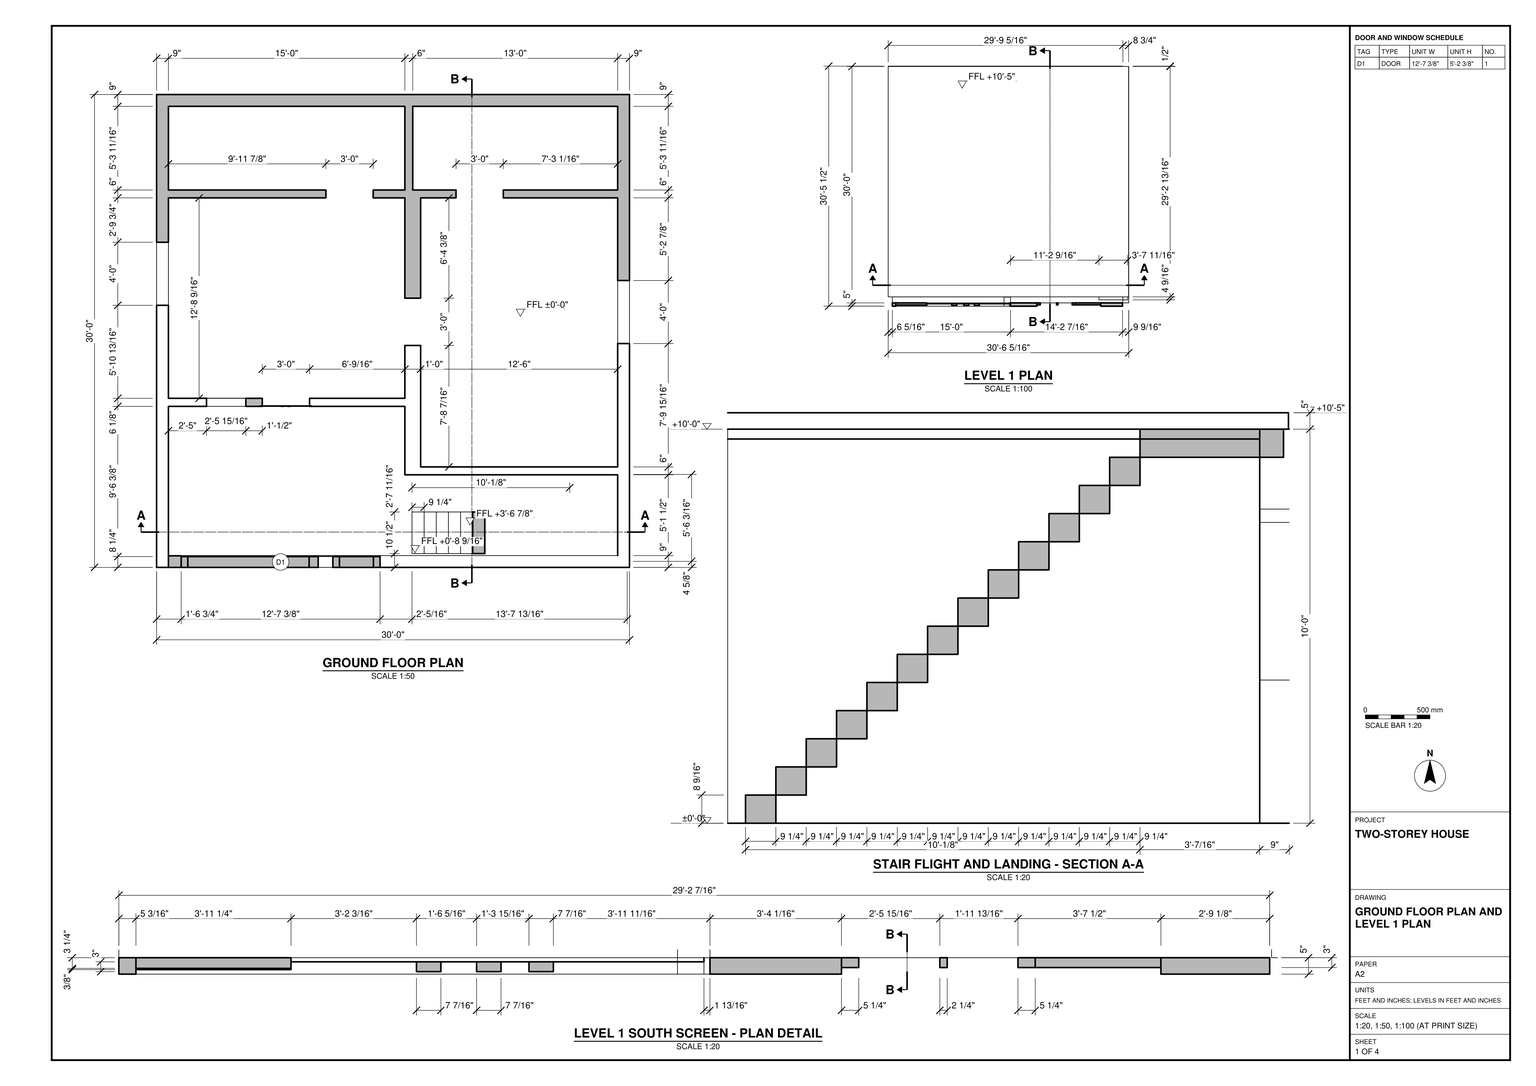
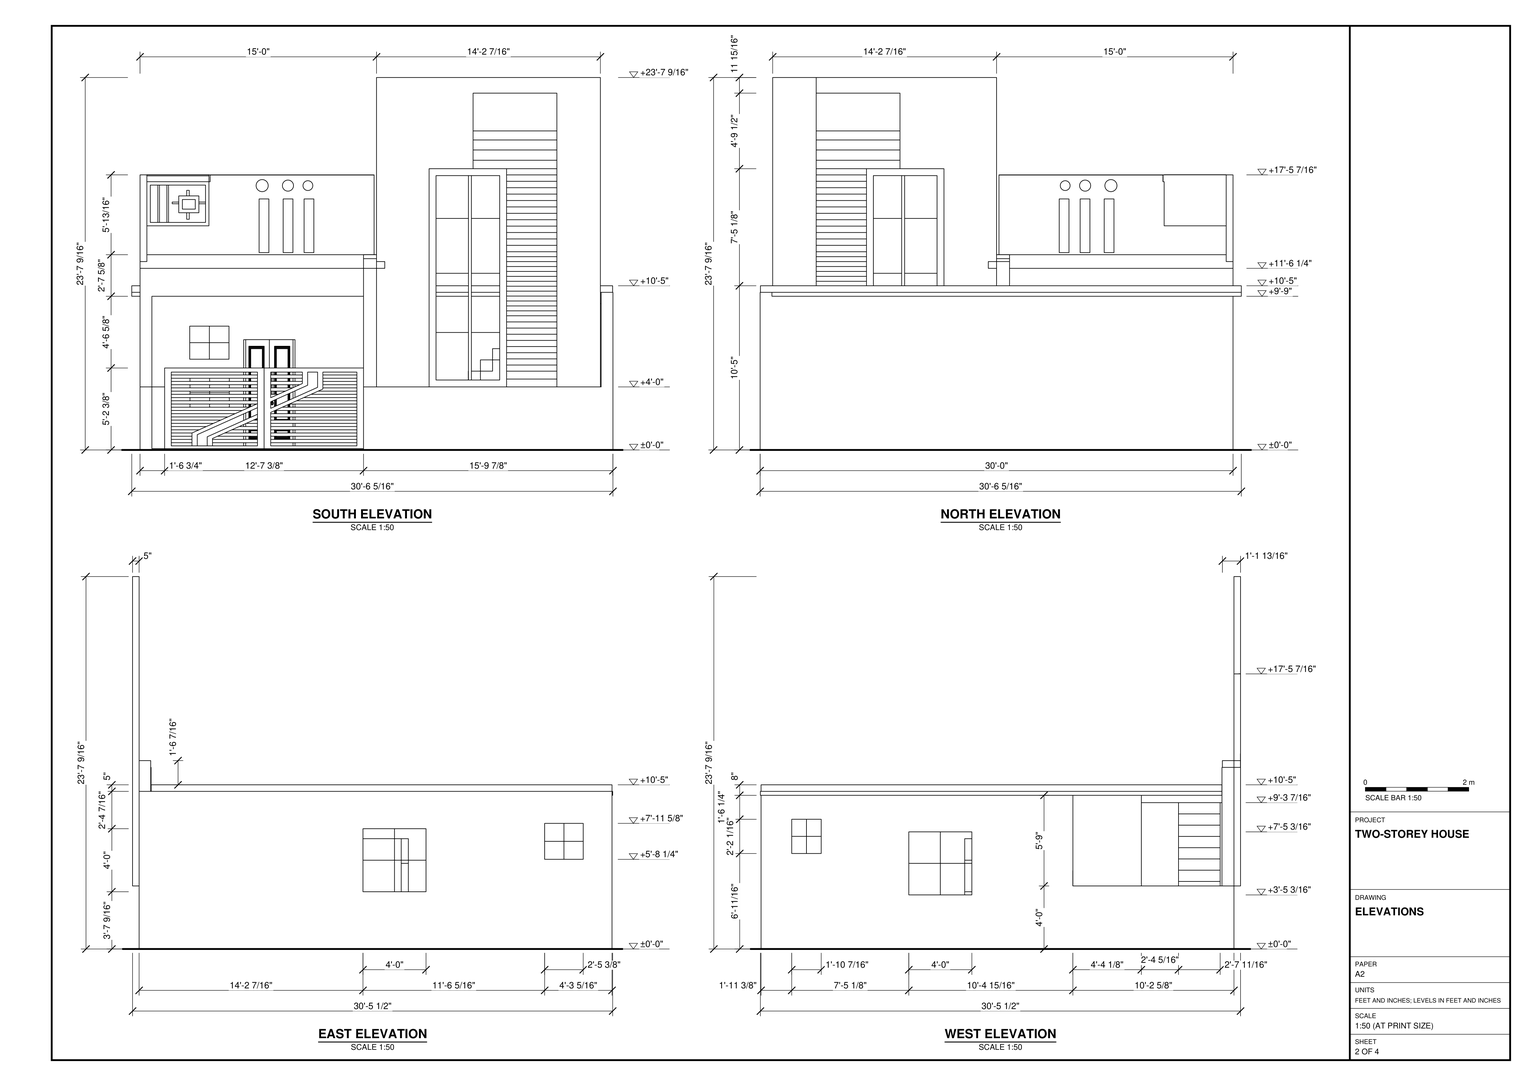
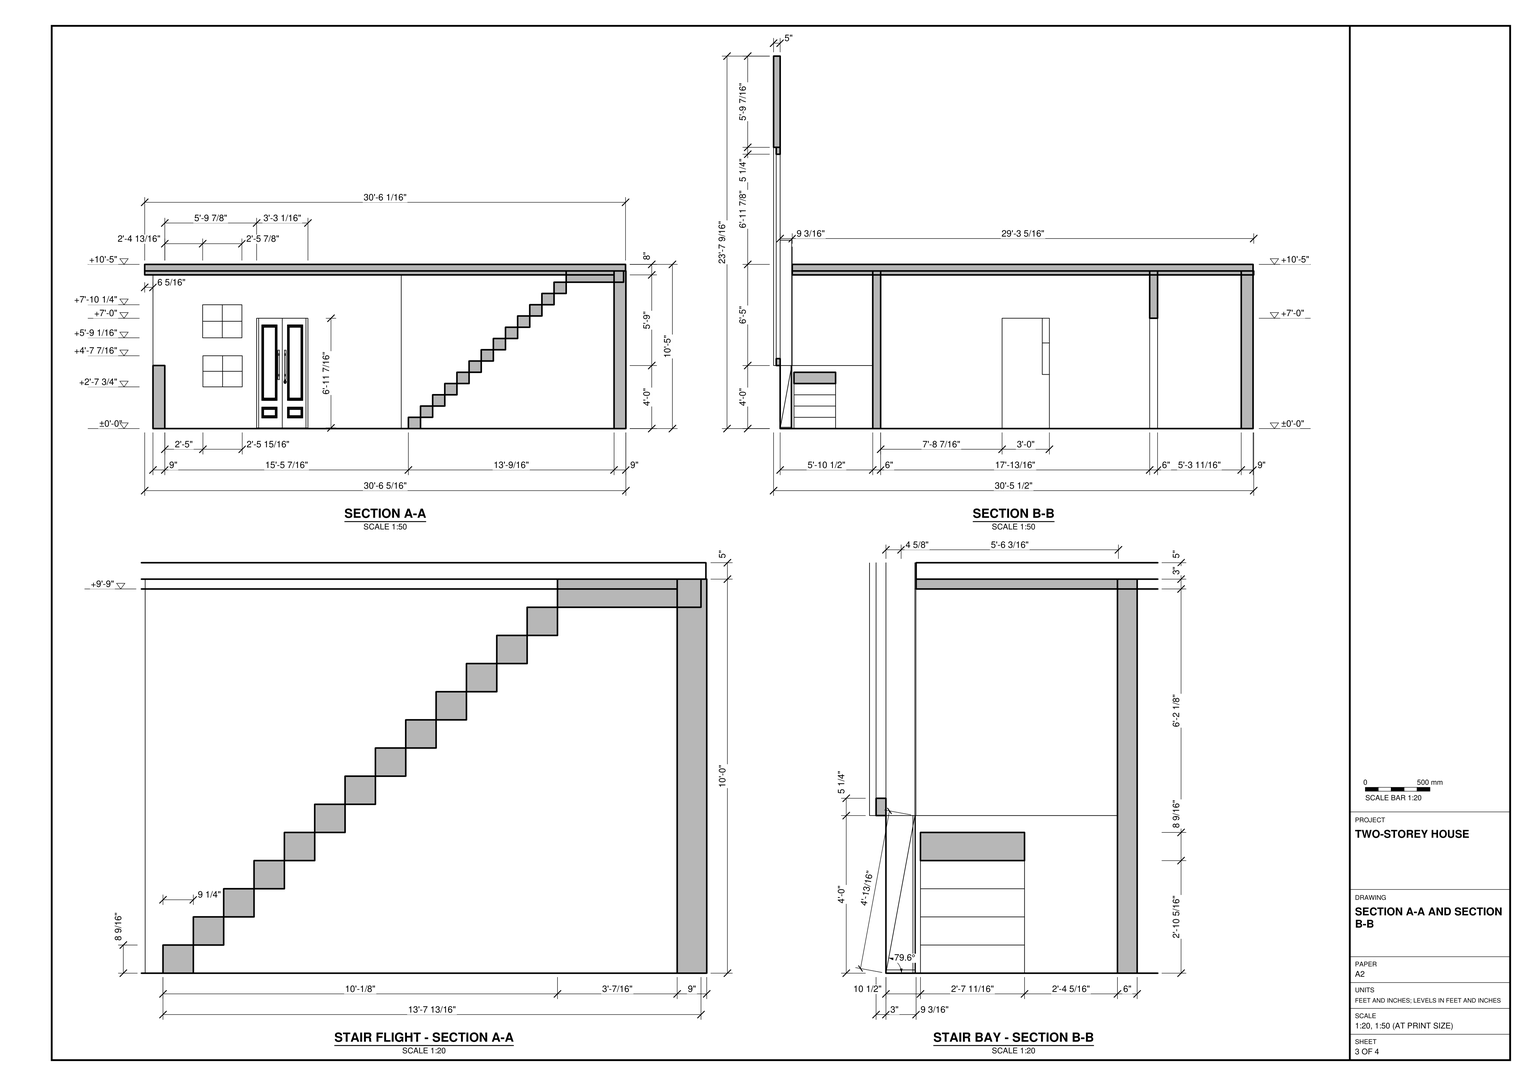
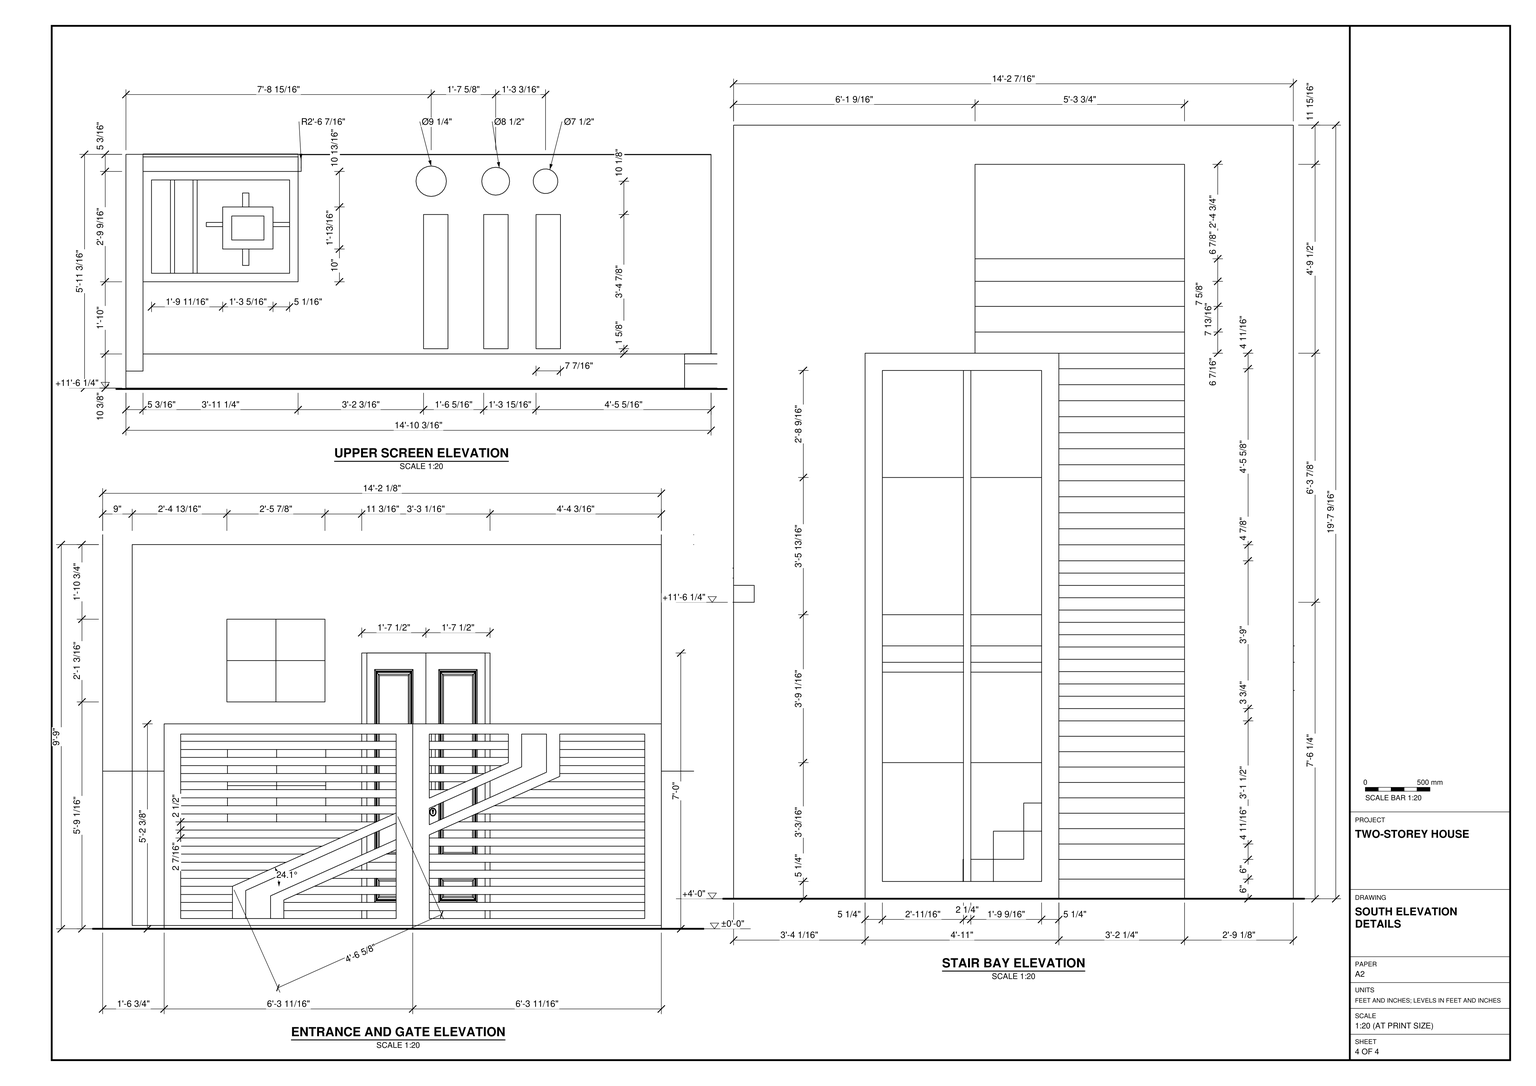
Build the house in SketchUp from task_files/diagram_01.pdf. Work in feet and inches. Orient the screened entrance toward the south. The overall model measures 30'-6 5/16" east to west, 30'-5 1/2" north to south and 23'-7 9/16" high. Set the ground floor at ±0'-0" and Level 1 at +10'-5".

Lay out the ground floor with the 9" exterior walls and 6" partitions shown in plan. Form the two rooms across the north end, the larger spaces south of them and the recessed entrance behind the front gate. Place the doorways and divided windows using the plan and elevations. Model the straight stair in the southeast bay, including its treads and upper landing. Use the sections to set the landing against the flat Level 1 slab and to shape the projecting slab edge.

Leave the upper slab open behind the south screen. Viewed from the south, the shorter panel sits over the gate on the left; the tall frame, horizontal bands and narrow divided panel stand on the right. Use the screen plan detail to place these elements at their different depths. Model the gate with its horizontal bars and diagonal motif.

Keep shell elements such as walls, slabs and roof, and each furniture or joinery piece shown, in separate groups or components; use components for repeated parts. Decor and loose items shown may be represented by any suitable library component. Save one SketchUp model as output_files/two_storey_house_with_a_stepped_south_screen.skp.

# SketchUp Ruby script. Lengths in inches.
U = 1.inch
M = Sketchup.active_model
def pt(a) = Geom::Point3d.new(a.map { |v| v * U })
def face(e, loops, mat)
  f = e.add_face(loops[0].map { |a| pt(a) })
  loops[1..].each { |l| e.add_face(l.map { |a| pt(a) }).erase! }
  f.material = f.back_material = mat if mat
  f
end
# faces: each face lists its corners as indices into pts; further lists are holes
def faces(e, pts, list, mat = nil) = list.each { |f| face(e, (f[0].is_a?(Array) ? f : [f]).map { |l| l.map { |i| pts[i] } }, mat) }
# xy, xz, yz: faces in a plane at the given z, y or x. An outline is a flat list of corners, or four numbers for a rectangle; further outlines are holes
def ring(l) = l.size == 4 ? [[l[0], l[1]], [l[2], l[1]], [l[2], l[3]], [l[0], l[3]]] : l.each_slice(2).to_a
def flat(e, list, mat, &to3) = list.each { |f| face(e, (f[0].is_a?(Array) ? f : [f]).map { |l| ring(l).map { |u, v| to3.(u, v) } }, mat) }
def xy(e, z, list, mat = nil) = flat(e, list, mat) { |x, y| [x, y, z] }
def xz(e, y, list, mat = nil) = flat(e, list, mat) { |x, z| [x, y, z] }
def yz(e, x, list, mat = nil) = flat(e, list, mat) { |y, z| [x, y, z] }
def lines(e, pts, list) = list.each { |a, b| e.add_line(pt(pts[a]), pt(pts[b])) }
# prism: a flat outline (further loops are holes) pulled along v
def prism(e, loops, v, mat = nil)
  f = face(e, loops, mat); d = Geom::Vector3d.new(v.map { |x| x * U })
  f.pushpull(f.normal.samedirection?(d) ? d.length : -d.length)
end
def box(e, o, s, mat = nil) = prism(e, [[o, [o[0] + s[0], o[1], o[2]], [o[0] + s[0], o[1] + s[1], o[2]], [o[0], o[1] + s[1], o[2]]]], [0, 0, s[2]], mat)
def at(x, y, z, deg = 0) = Geom::Transformation.translation(pt([x, y, z])) * Geom::Transformation.rotation(ORIGIN, Z_AXIS, deg.degrees)
def axes(o, x, y, z) = Geom::Transformation.new([*x, 0, *y, 0, *z, 0, *pt(o).to_a, 1])
def part(name) = M.definitions.add(name)
# library, detail: a bought-in or finely detailed component or shape, given as its bounding box
def library(name, o, s) = part(name).tap { |d| box(d.entities, o, s) }
def detail(e, o, s) = box(e.add_group.entities, o, s)
def put(e, d, t, mat = nil) = e.add_instance(d, t).tap { |i| i.material = mat if mat }
def group(e, t, mat = nil) = e.add_group.tap { |g| g.transformation = t; g.material = mat if mat }.entities
root = M.entities
M.materials.add("[Carrera Marble]").color = [207, 207, 207]
M.materials.add("[Color A08]").color = [102, 0, 0]
M.materials.add("[Color B04]").color = [255, 101, 50]
M.materials.add("[Color C06]").color = [204, 102, 0]
M.materials.add("[Color D06]").color = [204, 153, 0]
M.materials.add("[Color H06]").color = [0, 204, 204]
M.materials.add("[Color I02]").color = [153, 153, 255]
M.materials.add("[Color J02]").color = [204, 153, 255]
M.materials.add("[Color J03]").color = [178, 101, 255]
M.materials.add("[Color L02]").color = [255, 153, 204]
M.materials.add("[Color L04]").color = [255, 50, 152]
M.materials.add("[Color L11]").color = [153, 0, 76]
M.materials.add("[Color M04]").color = [142, 142, 142]
M.materials.add("[Color M06]").color = [86, 86, 86]
M.materials.add("[Color M08]").color = [30, 30, 30]
M.materials.add("[Concrete Aggregate Smoke]").color = [154, 150, 148]
M.materials.add("[Granite Light Gray]").color = [149, 148, 144]
M.materials.add("[Marble Carrara Gold Floor Tile]").color = [225, 223, 217]
M.materials.add("[Stone Vein Gray]").color = [166, 165, 165]
M.materials.add("[Translucent Glass Sky Reflection]").color = [126, 138, 183]
M.materials["[Translucent Glass Sky Reflection]"].alpha = 0.52
M.materials.add("[Wood Board Cork]").color = [215, 201, 115]
c1 = library("Modern+Gate+1",[-0.84,-7.98,-0.92],[117.88,7.98,57.34])
c2 = library("DD LT 2",[0,0,0],[47.24,4.7,78.74])
xy(root,0,[[[6.3125,5,6.3125,365,366.3125,365,366.3125,5,176.43,5,176.43,13.8125,25.03,13.8125,25.03,5],[15.3125,14,357.3125,14,357.3125,75.5,195.3125,75.5,195.3125,127.6,122.77,127.6,122.77,133.72,195.3125,133.72,195.3125,173.96,207.3125,173.96,207.3125,81.5,357.3125,81.5,357.3125,286.3125,270.25,286.3125,270.25,292.3125,357.3125,292.3125,357.3125,356,201.3125,356,201.3125,292.3125,234.25,292.3125,234.25,286.3125,207.3125,286.3125,207.3125,209.96,195.3125,209.96,195.3125,286.3125,171.2,286.3125,171.2,292.3125,195.3125,292.3125,195.3125,356,15.3125,356,15.3125,292.3125,135.2,292.3125,135.2,286.3125,15.3125,286.3125,15.3125,133.72,86.77,133.72,86.77,127.6,15.3125,127.6]],[25.03,5,176.43,13.8125]])
xy(root,0,[[15.3125,14,357.3125,14,357.3125,75.5,195.3125,75.5,195.3125,127.6,122.77,127.6,122.77,133.72,195.3125,133.72,195.3125,173.96,207.3125,173.96,207.3125,81.5,357.3125,81.5,357.3125,286.3125,270.25,286.3125,270.25,292.3125,357.3125,292.3125,357.3125,356,201.3125,356,201.3125,292.3125,234.25,292.3125,234.25,286.3125,207.3125,286.3125,207.3125,209.96,195.3125,209.96,195.3125,286.3125,171.2,286.3125,171.2,292.3125,195.3125,292.3125,195.3125,356,15.3125,356,15.3125,292.3125,135.2,292.3125,135.2,286.3125,15.3125,286.3125,15.3125,133.72,86.77,133.72,86.77,127.6,15.3125,127.6]],"[Marble Carrara Gold Floor Tile]")
xy(root,1,[[15.3125,5,25.03,13.8125],[25.03,5,176.43,13.8125]])
xy(root,31.75,[[44.32,127.6,74.26,133.72],[44.32,133.72,74.26,133.85]])
xy(root,41.19,[[6.3125,204.53,15.3125,252.53]])
xy(root,43.59,[[357.3125,175.41,366.3125,223.41]])
xy(root,48,[[186.3125,0,226.36,5],[323.625,0,356.75,5],[226.36,2,285.36,5],[285.36,2,323.625,5],[6.3125,5,15.3125,14.125],
  [15.3125,5,25.03,13.8125],[176.43,5,186.3125,13.8125]])
xy(root,48,[[6.3125,14.125,15.3125,127.6]],"[Color M08]")
xy(root,53.26,[[231.62,2,256.3,5],[256.3,2,258.55,5],[258.55,2,280.1,5]])
xy(root,53.97,[[285.36,2,323.625,5]],"[Color A08]")
xy(root,55.4375,[[44.32,127.6,74.26,133.72],[44.32,133.72,74.26,133.85]])
xy(root,59.97,[[285.36,5,323.625,8]])
xy(root,59.97,[[285.36,2,323.625,5]],"[Color A08]")
xy(root,64.66,[[285.36,5,323.625,8]])
xy(root,64.66,[[285.36,2,323.625,5]],"[Color A08]")
xy(root,68.28,[[357.3125,313.71,366.3125,343.08]])
xy(root,69.09,[[44.14,127.6,74.01,133.72]])
xy(root,69.35,[[285.36,2,323.625,5]],"[Color A08]")
xy(root,72.72,[[6.3125,319.21,15.3125,341.65]])
xy(root,74.04,[[285.36,2,323.625,5]],"[Color A08]")
xy(root,78.72,[[285.36,2,323.625,5]],"[Color A08]")
xy(root,83.41,[[285.36,2,323.625,5]],"[Color A08]")
xy(root,84,[[86.77,127.6,122.77,133.72],[195.3125,173.96,207.3125,209.96],[135.2,286.3125,171.2,292.3125],[234.25,286.3125,270.25,292.3125]])
xy(root,88.1,[[285.36,2,323.625,5]],"[Color A08]")
xy(root,89.19,[[6.3125,204.53,15.3125,252.53]])
xy(root,91.59,[[357.3125,175.41,366.3125,223.41]])
xy(root,92.79,[[285.36,2,323.625,5]],"[Color A08]")
xy(root,94.27,[[44.14,127.6,74.01,133.72]])
xy(root,95.65,[[357.3125,313.71,366.3125,343.08]])
xy(root,97.47,[[285.36,2,323.625,5]],"[Color A08]")
xy(root,98.78,[[6.3125,319.21,15.3125,341.65]])
xy(root,102.16,[[285.36,2,323.625,5]],"[Color A08]")
xy(root,105.91,[[285.36,2,323.625,5]],"[Color A08]")
xy(root,109.66,[[285.36,2,323.625,5]],"[Color A08]")
xy(root,113.41,[[285.36,2,323.625,5]],"[Color A08]")
xy(root,117,[[15.3125,5,176.43,14.125]])
xy(root,117.16,[[285.36,2,323.625,5]],"[Color A08]")
xy(root,120,[[[357.3125,5,366.3125,5,366.3125,365,6.3125,365,6.3125,127.6,195.3125,127.6,195.3125,75.5,357.3125,75.5],[207.3125,81.5,357.3125,286.3125],[15.3125,133.72,195.3125,286.3125],[15.3125,292.3125,195.3125,356],[201.3125,292.3125,357.3125,356]]])
xy(root,120.91,[[285.36,2,323.625,5]],"[Color A08]")
xy(root,124.66,[[285.36,2,323.625,5]],"[Color A08]")
xy(root,128.41,[[285.36,2,323.625,5]],"[Color A08]")
xy(root,132.16,[[285.36,2,323.625,5]],"[Color A08]")
xy(root,135.91,[[285.36,2,323.625,5]],"[Color A08]")
xy(root,138.27,[[186.3125,0,192.6,0.0625],[186.3125,0.0625,192.6,5]])
xy(root,138.27,[[6.3125,0,15.3125,5],[15.3125,0,176.43,5],[176.43,0,186.3125,5]],"[Color M06]")
xy(root,138.27,[[6.3125,5,176.43,14.125]],"[Concrete Aggregate Smoke]")
xy(root,139.66,[[285.36,2,323.625,5]],"[Color A08]")
xy(root,143.41,[[285.36,2,323.625,5]],"[Color A08]")
xy(root,143.4375,[[6.3125,0,11.52,5],[186.3125,0,189.6875,0.0625],[189.6875,0,192.6,0.0625],[186.3125,0.0625,189.6875,5],[189.6875,0.0625,192.6,5]])
xy(root,143.4375,[[176.43,5,186.3125,13.8125]],"[Concrete Aggregate Smoke]")
xy(root,145.64,[[176.43,0,186.3125,5]])
xy(root,147.16,[[285.36,2,323.625,5]],"[Color A08]")
xy(root,148.64,[[176.43,0,184.48,3.75],[176.43,3.75,184.48,5]])
xy(root,148.64,[[11.52,0,176.43,3.75]],"[Color M06]")
xy(root,148.71,[[176.43,0,186.3125,5]],"[Color M06]")
xy(root,150.25,[[96.94,0.75,104.38,3.75],[115.25,0.75,122.69,3.75],[131.19,0.75,138.63,3.75]],"[Color L04]")
xy(root,150.91,[[285.36,2,323.625,5]],"[Color A08]")
xy(root,155.79,[[285.36,2,323.625,5]],"[Color A08]")
xy(root,160.66,[[285.36,2,323.625,5]],"[Color A08]")
xy(root,165.54,[[285.36,2,323.625,5]],"[Color A08]")
xy(root,170.41,[[285.36,2,323.625,5]],"[Color A08]")
xy(root,170.64,[[11.52,1.375,58.74,1.75],[11.52,1.75,58.74,3.75],[11.52,3.75,58.74,5]])
xy(root,173.22,[[14.1,1.375,56.16,1.75]])
xy(root,173.22,[[14.1,1.75,56.16,1.75,56.16,3.75,28,3.75,28,1.875,26.75,1.875,26.75,3.75,21.125,3.75,21.125,2.0625,19.87,2.0625,19.87,3.75,14.1,3.75]],"[Color M04]")
xy(root,175.29,[[285.36,2,323.625,5]],"[Color A08]")
xy(root,175.61,[[41.83,1.75,43.77,3.75]],"[Color M08]")
xy(root,180.16,[[285.36,2,323.625,5]],"[Color A08]")
xy(root,180.61,[[41.83,1.75,43.77,3.75]])
xy(root,180.61,[[35.78,1.75,41.83,3.75],[43.77,1.75,51.1,3.75]],"[Color C06]")
xy(root,183.36,[[38.54,1.75,48.34,3.6875],[38.54,3.6875,48.34,3.75],[38.54,3.75,48.34,4.625]])
xy(root,183.36,[[38.54,0.6875,48.34,1.75]],"[Color D06]")
xy(root,185.04,[[285.36,2,323.625,5]],"[Color A08]")
xy(root,187.43,[[30.78,1.75,35.78,3.75],[51.1,1.75,56.16,3.75]],"[Color M08]")
xy(root,188.71,[[30.78,1.75,35.78,3.75],[51.1,1.75,56.16,3.75]],"[Color M08]")
xy(root,189.91,[[285.36,2,323.625,5]],"[Color A08]")
xy(root,190.67,[[38.54,1.75,48.34,3.6875],[38.54,3.6875,48.34,3.75],[38.54,3.75,48.34,4.625]])
xy(root,190.67,[[38.54,0.6875,48.34,1.75]],"[Color D06]")
xy(root,191.12,[[131.19,0.75,138.63,3.75]])
xy(root,191.12,[[96.94,0.75,104.38,3.75],[115.25,0.75,122.69,3.75]],"[Color L04]")
xy(root,193.42,[[41.83,1.75,43.77,3.75]])
xy(root,193.42,[[35.78,1.75,41.83,3.75],[43.77,1.75,51.1,3.75]],"[Color C06]")
xy(root,194.79,[[285.36,2,323.625,5]],"[Color A08]")
xy(root,197.67,[[41.83,1.75,43.77,3.75]],"[Color M08]")
xy(root,199.66,[[285.36,2,323.625,5]],"[Color A08]")
xy(root,201.65,[[14.1,1.375,56.16,1.75]])
xy(root,201.65,[[14.1,1.75,14.1,3.75,19.87,3.75,19.87,2.0625,21.125,2.0625,21.125,3.75,26.75,3.75,26.75,1.875,28,1.875,28,3.75,56.16,3.75,56.16,1.75]],"[Color M04]")
xy(root,204.23,[[11.52,1.375,58.74,1.75],[58.74,3.75,59.54,5]])
xy(root,204.23,[[11.52,0,58.74,1.375],[58.74,0,58.74,3.75,59.54,3.75,59.68,0]],"[Color M06]")
xy(root,204.54,[[285.36,2,323.625,5]],"[Color A08]")
xy(root,208.67,[[11.52,0,58.74,1.375]])
xy(root,208.87,[[231.62,2,256.3,5],[256.3,2,258.55,5],[258.55,2,280.1,5]])
xy(root,209.3125,[[59.68,3.75,184.48,5]])
xy(root,209.41,[[285.36,2,323.625,5]],"[Color A08]")
xy(root,209.4375,[[59.68,0,59.68,3.75,59.54,3.75],[59.54,3.75,59.68,5],[59.68,3.75,184.48,5]])
xy(root,209.4375,[[6.3125,0,11.52,5],[11.52,1.375,58.74,1.375,58.74,3.75,59.54,3.75,59.54,5,11.52,5]],"[Color M06]")
xy(root,209.48,[[11.52,0,58.74,1.375]])
xy(root,209.54,[[11.52,0,58.74,1.375]],"[Color M06]")
xy(root,214.125,[[226.36,0,259.83,2],[226.36,2,259.83,5]])
xy(root,214.125,[[259.83,2,285.36,5],[285.36,2,323.625,5]],"[Color A08]")
xy(root,220.57,[[259.83,2,323.625,5]],"[Color A08]")
xy(root,228.38,[[259.83,2,323.625,5]],"[Color A08]")
xy(root,236.01,[[259.83,2,323.625,5]],"[Color A08]")
xy(root,242.88,[[259.83,2,323.625,5]],"[Color A08]")
xy(root,271.64,[[259.83,0,323.625,5]])
xy(root,283.5625,[[186.3125,0,356.75,5]],"[Color H06]")
xz(root,0,[[176.43,148.64,186.3125,148.71],[11.52,209.4375,58.74,209.48],[11.52,209.48,58.74,209.54]])
xz(root,0,[[186.3125,48,226.36,48,226.36,214.125,259.83,214.125,259.83,271.64,323.625,271.64,323.625,48,356.75,48,356.75,283.5625,186.3125,283.5625,186.3125,143.4375,192.6,143.4375,192.6,138.27,186.3125,138.27]],"[Color H06]")
xz(root,0,[[6.3125,138.27,176.43,138.27,176.43,148.64,11.52,148.64,11.52,143.4375,6.3125,143.4375],[176.43,138.27,186.3125,145.64],[6.3125,143.4375,11.52,209.4375],[176.43,145.64,186.3125,148.64],[11.52,204.23,58.74,208.67],
  [58.74,204.23,59.68,209.4375],[11.52,208.67,58.74,209.4375]],"[Color M06]")
xz(root,0.0625,[[186.3125,138.27,192.6,143.4375]],"[Color H06]")
xz(root,0.6875,[[38.54,183.36,48.34,190.67]],"[Color D06]")
xz(root,0.75,[[96.94,150.25,104.38,191.12],[115.25,150.25,122.69,191.12],[131.19,150.25,138.63,191.12]],"[Color L04]")
xz(root,0.75,[[99.27,196.63,100.46,196.79,101.58,197.25,102.54,197.99,103.27,198.95,103.73,200.0625,103.89,201.26,103.73,202.45,103.27,203.57,102.54,204.53,101.58,205.26,100.46,205.73,99.27,205.88,98.07,205.73,96.96,205.26,96,204.53,95.26,203.57,94.8,202.45,94.64,201.26,94.8,200.0625,95.26,198.95,96,197.99,96.96,197.25,98.07,196.79],[118.9,197.02,120,197.16,121.02,197.59,121.9,198.26,122.57,199.14,123,200.16,123.14,201.26,123,202.35,122.57,203.38,121.9,204.26,121.02,204.93,120,205.35,118.9,205.5,117.8,205.35,116.78,204.93,115.9,204.26,115.23,203.38,114.81,202.35,114.66,201.26,114.81,200.16,115.23,199.14,115.9,198.26,116.78,197.59,117.8,197.16],[133.73,197.52,134.71,197.5625,135.64,197.85,136.47,198.37,137.14,199.09,137.6,199.95,137.8125,200.91,137.78,201.89,137.49,202.82,136.97,203.65,136.25,204.32,135.38,204.77,134.43,204.99,133.45,204.95,132.52,204.67,131.6875,204.15,131.02,203.43,130.5625,202.5625,130.35,201.61,130.38,200.63,130.67,199.69,131.19,198.87,131.91,198.2,132.78,197.74]],"[Color M06]")
xz(root,1.375,[[11.52,204.23,58.74,208.67],[11.52,208.67,58.74,209.4375],[11.52,209.4375,58.74,209.48],[11.52,209.48,58.74,209.54]])
xz(root,1.375,[[[11.52,170.64,58.74,204.23],[14.1,173.22,56.16,201.65]]],"[Color M04]")
xz(root,1.75,[[[11.52,170.64,58.74,204.23],[14.1,173.22,56.16,201.65]]])
xz(root,1.75,[[[35.78,180.61,51.1,193.42],[38.54,183.36,48.34,190.67]]],"[Color C06]")
xz(root,1.75,[[41.83,175.61,43.77,180.61],[30.78,187.43,35.78,188.71],[51.1,187.43,56.16,188.71],[41.83,193.42,43.77,197.67]],"[Color M08]")
xz(root,1.875,[[26.75,173.22,28,201.65]],"[Color L02]")
xz(root,2,[[285.36,48,323.625,53.97],[285.36,59.97,323.625,64.66],[285.36,69.35,323.625,74.04],[285.36,78.72,323.625,83.41],[285.36,88.1,323.625,92.79],
  [285.36,97.47,323.625,102.16],[285.36,105.91,323.625,109.66],[285.36,113.41,323.625,117.16],[285.36,120.91,323.625,124.66],[285.36,128.41,323.625,132.16],
  [285.36,135.91,323.625,139.66],[285.36,143.41,323.625,147.16],[285.36,150.91,323.625,155.79],[285.36,160.66,323.625,165.54],[285.36,170.41,323.625,175.29],
  [285.36,180.16,323.625,185.04],[285.36,189.91,323.625,194.79],[285.36,199.66,323.625,204.54],[285.36,209.41,323.625,214.125],[259.83,220.57,323.625,228.38],
  [259.83,236.01,323.625,242.88]],"[Color A08]")
xz(root,2,[[[226.36,48,285.36,214.125],[231.62,53.26,280.1,208.87]]],"[Color I02]")
xz(root,2,[[256.3,53.26,258.55,208.87]],"[Color L11]")
xz(root,2.0625,[[19.87,173.22,21.125,201.65]],"[Color L02]")
xz(root,3.6875,[[38.54,183.36,48.34,190.67]])
xz(root,3.75,[[96.94,150.25,104.38,191.12],[115.25,150.25,122.69,191.12],[131.19,150.25,138.63,191.12],[41.83,175.61,43.77,180.61],[[35.78,180.61,35.78,193.42,41.83,193.42,41.83,192.67,43.77,192.67,43.77,193.42,51.1,193.42,51.1,180.61],[38.54,183.36,48.34,190.67]],
  [38.54,183.36,48.34,190.67],[30.78,187.43,35.78,188.71],[41.83,192.67,43.77,193.42],[41.83,193.42,43.77,197.67],[59.68,209.3125,184.48,209.4375]])
xz(root,3.75,[[14.1,173.22,19.87,201.65],[21.125,173.22,26.75,201.65],[[28,173.22,56.16,173.22,56.16,187.43,51.1,187.43,51.1,180.61,43.77,180.61,43.77,175.61,41.83,175.61,41.83,180.61,35.78,180.61,35.78,187.43,30.78,187.43,30.78,188.71,35.78,188.71,35.78,193.42,51.1,193.42,51.1,188.71,56.16,188.71,56.16,201.65,28,201.65],[41.83,192.67,43.77,197.67]]],"[Color B04]")
xz(root,3.75,[[58.74,204.23,59.54,209.4375]],"[Color M06]")
xz(root,3.75,[[[11.52,148.64,184.48,148.64,184.48,209.3125,59.68,209.3125,59.68,209.4375,59.54,209.4375,59.54,204.23,58.74,204.23,58.74,170.64,11.52,170.64],[96.94,150.25,104.38,191.12],[115.25,150.25,122.69,191.12],[131.19,150.25,138.63,191.12],[99.27,196.63,98.07,196.79,96.96,197.25,96,197.99,95.26,198.95,94.8,200.0625,94.64,201.26,94.8,202.45,95.26,203.57,96,204.53,96.96,205.26,98.07,205.73,99.27,205.88,100.46,205.73,101.58,205.26,102.54,204.53,103.27,203.57,103.73,202.45,103.89,201.26,103.73,200.0625,103.27,198.95,102.54,197.99,101.58,197.25,100.46,196.79],[118.9,197.02,117.8,197.16,116.78,197.59,115.9,198.26,115.23,199.14,114.81,200.16,114.66,201.26,114.81,202.35,115.23,203.38,115.9,204.26,116.78,204.93,117.8,205.35,118.9,205.5,120,205.35,121.02,204.93,121.9,204.26,122.57,203.38,123,202.35,123.14,201.26,123,200.16,122.57,199.14,121.9,198.26,121.02,197.59,120,197.16],[133.73,197.52,132.78,197.74,131.91,198.2,131.19,198.87,130.67,199.69,130.38,200.63,130.35,201.61,130.5625,202.5625,131.02,203.43,131.6875,204.15,132.52,204.67,133.45,204.95,134.43,204.99,135.38,204.77,136.25,204.32,136.97,203.65,137.49,202.82,137.78,201.89,137.8125,200.91,137.6,199.95,137.14,199.09,136.47,198.37,135.64,197.85,134.71,197.5625]]],"[Granite Light Gray]")
xz(root,4.625,[[38.54,183.36,48.34,190.67]])
xz(root,5,[[25.03,0,176.43,1],[186.3125,48,186.3125,138.27,192.6,138.27,192.6,143.4375,186.3125,143.4375,186.3125,283.5625,323.625,283.5625,323.625,271.64,259.83,271.64,259.83,214.125,226.36,214.125,226.36,48],[[226.36,48,285.36,214.125],[231.62,53.26,280.1,208.87]],[285.36,48,323.625,53.97],[323.625,48,356.75,283.5625],
  [256.3,53.26,258.55,208.87],[285.36,59.97,323.625,64.66],[285.36,69.35,323.625,74.04],[285.36,78.72,323.625,83.41],[285.36,88.1,323.625,92.79],
  [285.36,97.47,323.625,102.16],[285.36,105.91,323.625,109.66],[285.36,113.41,323.625,117.16],[285.36,120.91,323.625,124.66],[285.36,128.41,323.625,132.16],
  [285.36,135.91,323.625,139.66],[176.43,138.27,186.3125,143.4375],[186.3125,138.27,192.6,143.4375],[285.36,143.41,323.625,147.16],[176.43,143.4375,186.3125,145.64],
  [176.43,145.64,186.3125,148.64],[176.43,148.64,184.48,148.71],[184.48,148.64,186.3125,148.71],[285.36,150.91,323.625,155.79],[285.36,160.66,323.625,165.54],
  [285.36,170.41,323.625,175.29],[285.36,180.16,323.625,185.04],[285.36,189.91,323.625,194.79],[285.36,199.66,323.625,204.54],[59.68,209.3125,184.48,209.4375],
  [285.36,209.41,323.625,214.125]])
xz(root,5,[[6.3125,48,15.3125,48,15.3125,117,176.43,117,176.43,138.27,6.3125,138.27],[176.43,48,186.3125,138.27]],"[Color J02]")
xz(root,5,[[6.3125,0,25.03,0,25.03,1,15.3125,1,15.3125,48,6.3125,48],[176.43,0,366.3125,0,366.3125,120,357.3125,120,357.3125,48,176.43,48],[15.3125,1,25.03,48]],"[Color M08]")
xz(root,5,[[6.3125,138.27,6.3125,143.4375,11.52,143.4375,11.52,148.64,176.43,148.64,176.43,138.27],[6.3125,143.4375,11.52,209.4375],[11.52,170.64,11.52,209.4375,59.54,209.4375,59.54,204.23,58.74,204.23,58.74,170.64]],"[Concrete Aggregate Smoke]")
xz(root,5,[[285.36,53.97,323.625,59.97],[285.36,64.66,323.625,69.35],[285.36,74.04,323.625,78.72],[285.36,83.41,323.625,88.1],[285.36,92.79,323.625,97.47],
  [285.36,102.16,323.625,105.91],[285.36,109.66,323.625,113.41],[285.36,117.16,323.625,120.91],[285.36,124.66,323.625,128.41],[285.36,132.16,323.625,135.91],
  [285.36,139.66,323.625,143.41],[285.36,147.16,323.625,150.91],[285.36,155.79,323.625,160.66],[285.36,165.54,323.625,170.41],[285.36,175.29,323.625,180.16],
  [285.36,185.04,323.625,189.91],[285.36,194.79,323.625,199.66],[285.36,204.54,323.625,209.41],[259.83,214.125,323.625,220.57],[259.83,228.38,323.625,236.01]],"[Wood Board Cork]")
xz(root,8,[[285.36,59.97,323.625,64.66]])
xz(root,13.8125,[[25.03,0,176.43,1],[15.3125,1,25.03,48]])
xz(root,13.8125,[[176.43,48,186.3125,143.4375]],"[Concrete Aggregate Smoke]")
xz(root,14.125,[[6.3125,48,6.3125,138.27,176.43,138.27,176.43,117,15.3125,117,15.3125,48]],"[Concrete Aggregate Smoke]")
xz(root,75.5,[[195.3125,0,357.3125,120]],"[Stone Vein Gray]")
xz(root,81.5,[[207.3125,0,357.3125,120]])
xz(root,127.6,[[[15.3125,0,86.77,0,86.77,84,122.77,84,122.77,0,195.3125,0,195.3125,120,6.3125,120,6.3125,48,15.3125,48],[44.14,69.09,74.01,94.27],[44.32,31.75,74.26,55.4375]]],"[Stone Vein Gray]")
xz(root,133.72,[[[15.3125,0,86.77,0,86.77,84,122.77,84,122.77,0,195.3125,0,195.3125,120,15.3125,120],[44.14,69.09,74.01,94.27],[44.32,31.75,74.26,55.4375]]])
xz(root,173.96,[[195.3125,0,207.3125,84]])
xz(root,175.41,[[357.3125,43.59,366.3125,91.59]])
xz(root,204.53,[[6.3125,41.19,15.3125,89.19]])
xz(root,209.96,[[195.3125,0,207.3125,84]])
xz(root,223.41,[[357.3125,43.59,366.3125,91.59]])
xz(root,252.53,[[6.3125,41.19,15.3125,89.19]])
xz(root,286.3125,[[207.3125,0,234.25,0,234.25,84,270.25,84,270.25,0,357.3125,0,357.3125,120,207.3125,120]])
xz(root,286.3125,[[15.3125,0,135.2,0,135.2,84,171.2,84,171.2,0,195.3125,0,195.3125,120,15.3125,120]],"[Translucent Glass Sky Reflection]")
xz(root,292.3125,[[15.3125,0,15.3125,120,195.3125,120,195.3125,0,171.2,0,171.2,84,135.2,84,135.2,0],[201.3125,0,201.3125,120,357.3125,120,357.3125,0,270.25,0,270.25,84,234.25,84,234.25,0]])
xz(root,313.71,[[357.3125,68.28,366.3125,95.65]])
xz(root,319.21,[[6.3125,72.72,15.3125,98.78]])
xz(root,341.65,[[6.3125,72.72,15.3125,98.78]])
xz(root,343.08,[[357.3125,68.28,366.3125,95.65]])
xz(root,356,[[15.3125,0,195.3125,120],[201.3125,0,357.3125,120]])
xz(root,365,[[6.3125,0,366.3125,120]],"[Color M08]")
yz(root,6.3125,[[5,48,14.125,138.27]],"[Color J03]")
yz(root,6.3125,[[[5,0,5,48,127.6,48,127.6,120,365,120,365,0],[204.53,41.19,252.53,89.19],[319.21,72.72,341.65,98.78]]],"[Color M08]")
yz(root,6.3125,[[0,138.27,5,143.4375],[0,143.4375,5,209.4375]],"[Concrete Aggregate Smoke]")
yz(root,11.52,[[0,143.4375,5,148.64],[3.75,148.64,5,170.64],[1.375,170.64,1.75,204.23],[1.75,170.64,5,170.64,5,209.4375,1.375,209.4375,1.375,204.23,1.75,204.23],[0,204.23,1.375,208.67],
  [0,208.67,1.375,209.4375],[0,209.4375,1.375,209.48],[0,209.48,1.375,209.54]])
yz(root,11.52,[[0,148.64,0,204.23,1.375,204.23,1.375,170.64,3.75,170.64,3.75,148.64]],"[Color M06]")
yz(root,14.1,[[1.375,173.22,1.75,201.65]])
yz(root,14.1,[[1.75,173.22,3.75,201.65]],"[Color M04]")
yz(root,15.3125,[[[133.72,0,286.3125,120],[204.53,41.19,252.53,89.19]],[[292.3125,0,356,120],[319.21,72.72,341.65,98.78]],[5,1,13.8125,48],[5,48,14.125,117]])
yz(root,15.3125,[[14,0,127.6,48]],"[Color M08]")
yz(root,19.87,[[2.0625,173.22,3.75,201.65]],"[Color L02]")
yz(root,21.125,[[2.0625,173.22,3.75,201.65]],"[Color L02]")
yz(root,25.03,[[5,0,13.8125,1],[5,1,13.8125,48]])
yz(root,26.75,[[1.875,173.22,3.75,201.65]],"[Color L02]")
yz(root,28,[[1.875,173.22,3.75,201.65]],"[Color L02]")
yz(root,30.78,[[1.75,187.43,3.75,188.71]],"[Color M08]")
yz(root,35.78,[[1.75,187.43,3.75,188.71]])
yz(root,35.78,[[1.75,180.61,3.75,187.43],[1.75,188.71,3.75,193.42]],"[Color C06]")
yz(root,38.54,[[1.75,183.36,3.6875,190.67],[3.6875,183.36,3.75,190.67],[3.75,183.36,4.625,190.67]])
yz(root,38.54,[[0.6875,183.36,1.75,190.67]],"[Color D06]")
yz(root,41.83,[[1.75,175.61,3.75,180.61],[1.75,193.42,3.75,197.67]],"[Color M08]")
yz(root,43.77,[[1.75,175.61,3.75,180.61],[1.75,193.42,3.75,197.67]],"[Color M08]")
yz(root,44.14,[[127.6,69.09,133.72,94.27]])
yz(root,44.32,[[127.6,31.75,133.72,55.4375],[133.72,31.75,133.85,55.4375]])
yz(root,48.34,[[1.75,183.36,3.6875,190.67],[3.6875,183.36,3.75,190.67],[3.75,183.36,4.625,190.67]])
yz(root,48.34,[[0.6875,183.36,1.75,190.67]],"[Color D06]")
yz(root,51.1,[[1.75,187.43,3.75,188.71]])
yz(root,51.1,[[1.75,180.61,3.75,187.43],[1.75,188.71,3.75,193.42]],"[Color C06]")
yz(root,56.16,[[1.375,173.22,1.75,187.43],[1.75,173.22,3.75,187.43],[1.375,187.43,1.75,188.71],[1.375,188.71,1.75,201.65],[1.75,188.71,3.75,201.65]],"[Color M04]")
yz(root,58.74,[[1.375,170.64,1.75,204.23],[1.75,170.64,3.75,204.23],[3.75,170.64,5,204.23],[0,204.23,1.375,208.67],[1.375,204.23,3.75,209.4375],
  [0,208.67,1.375,209.4375],[0,209.4375,1.375,209.48],[0,209.48,1.375,209.54]])
yz(root,59.54,[[3.75,204.23,5,209.4375]])
yz(root,59.68,[[3.75,209.3125,5,209.4375]])
yz(root,74.01,[[127.6,69.09,133.72,94.27]])
yz(root,74.26,[[127.6,31.75,133.72,55.4375],[133.72,31.75,133.85,55.4375]])
yz(root,86.77,[[127.6,0,133.72,84]])
yz(root,96.94,[[0.75,150.25,3.75,191.12]],"[Color L04]")
yz(root,104.38,[[0.75,150.25,3.75,191.12]],"[Color L04]")
yz(root,115.25,[[0.75,150.25,3.75,191.12]],"[Color L04]")
yz(root,122.69,[[0.75,150.25,3.75,191.12]],"[Color L04]")
yz(root,122.77,[[127.6,0,133.72,84]])
yz(root,131.19,[[0.75,150.25,3.75,191.12]],"[Color L04]")
yz(root,135.2,[[286.3125,0,292.3125,84]])
yz(root,138.63,[[0.75,150.25,3.75,191.12]],"[Color L04]")
yz(root,171.2,[[286.3125,0,292.3125,84]])
yz(root,176.43,[[5,0,5.18,1,13.8125,1,13.8125,0],[5,0,5.18,1,5,1],[5,1,5,48,13.8125,48,5.18,1],[5.18,1,13.8125,48,13.8125,1],[5,48,13.8125,117],
  [5,117,13.8125,138.27],[13.8125,117,14.125,138.27],[0,138.27,5,145.64],[0,145.64,5,148.64],[0,148.64,5,148.71]])
yz(root,176.43,[[5,138.27,13.8125,143.4375]],"[Concrete Aggregate Smoke]")
yz(root,184.48,[[3.75,148.64,5,209.3125],[3.75,209.3125,5,209.4375]])
yz(root,186.3125,[[5,48,13.8125,143.4375],[0,138.27,0.0625,143.4375],[0.0625,138.27,5,143.4375],[0,143.4375,0.0625,145.64],[0.0625,143.4375,5,145.64],
  [0,145.64,0.0625,148.64],[0.0625,145.64,5,148.64],[0,148.64,0.0625,148.71],[0.0625,148.64,5,148.71]])
yz(root,186.3125,[[0,48,5,138.27],[0,148.71,5,283.5625]],"[Color H06]")
yz(root,192.6,[[0,138.27,0.0625,143.4375],[0.0625,138.27,5,143.4375]])
yz(root,195.3125,[[133.72,0,133.72,120,286.3125,120,286.3125,0,209.96,0,209.96,84,173.96,84,173.96,0],[292.3125,0,356,120]])
yz(root,195.3125,[[75.5,0,127.6,120]],"[Stone Vein Gray]")
yz(root,201.3125,[[292.3125,0,356,120]])
yz(root,207.3125,[[81.5,0,173.96,0,173.96,84,209.96,84,209.96,0,286.3125,0,286.3125,120,81.5,120]])
yz(root,226.36,[[2,48,5,214.125]])
yz(root,226.36,[[0,48,2,214.125]],"[Color H06]")
yz(root,231.62,[[2,53.26,5,208.87]],"[Color I02]")
yz(root,234.25,[[286.3125,0,292.3125,84]])
yz(root,256.3,[[2,53.26,5,208.87]],"[Color L11]")
yz(root,258.55,[[2,53.26,5,208.87]],"[Color L11]")
yz(root,259.83,[[2,220.57,5,228.38],[2,236.01,5,242.88]])
yz(root,259.83,[[0,214.125,5,214.125,5,220.57,2,220.57,2,228.38,5,228.38,5,236.01,2,236.01,2,242.88,5,242.88,5,271.64,0,271.64]],"[Color H06]")
yz(root,270.25,[[286.3125,0,292.3125,84]])
yz(root,280.1,[[2,53.26,5,208.87]],"[Color I02]")
yz(root,285.36,[[2,48,5,53.97],[2,53.97,5,59.97],[2,59.97,5,64.66],[5,59.97,8,64.66],[2,64.66,5,69.35],
  [2,69.35,5,74.04],[2,74.04,5,78.72],[2,78.72,5,83.41],[2,83.41,5,88.1],[2,88.1,5,92.79],
  [2,92.79,5,97.47],[2,97.47,5,102.16],[2,102.16,5,105.91],[2,105.91,5,109.66],[2,109.66,5,113.41],
  [2,113.41,5,117.16],[2,117.16,5,120.91],[2,120.91,5,124.66],[2,124.66,5,128.41],[2,128.41,5,132.16],
  [2,132.16,5,135.91],[2,135.91,5,139.66],[2,139.66,5,143.41],[2,143.41,5,147.16],[2,147.16,5,150.91],
  [2,150.91,5,155.79],[2,155.79,5,160.66],[2,160.66,5,165.54],[2,165.54,5,170.41],[2,170.41,5,175.29],
  [2,175.29,5,180.16],[2,180.16,5,185.04],[2,185.04,5,189.91],[2,189.91,5,194.79],[2,194.79,5,199.66],
  [2,199.66,5,204.54],[2,204.54,5,209.41],[2,209.41,5,214.125]])
yz(root,323.625,[[0,48,0,271.64,5,271.64,5,242.88,2,242.88,2,236.01,5,236.01,5,228.38,2,228.38,2,220.57,5,220.57,5,214.125,2,214.125,2,209.41,5,209.41,5,204.54,2,204.54,2,199.66,5,199.66,5,194.79,2,194.79,2,189.91,5,189.91,5,185.04,2,185.04,2,180.16,5,180.16,5,175.29,2,175.29,2,170.41,5,170.41,5,165.54,2,165.54,2,160.66,5,160.66,5,155.79,2,155.79,2,150.91,5,150.91,5,147.16,2,147.16,2,143.41,5,143.41,5,139.66,2,139.66,2,135.91,5,135.91,5,132.16,2,132.16,2,128.41,5,128.41,5,124.66,2,124.66,2,120.91,5,120.91,5,117.16,2,117.16,2,113.41,5,113.41,5,109.66,2,109.66,2,105.91,5,105.91,5,102.16,2,102.16,2,97.47,5,97.47,5,92.79,2,92.79,2,88.1,5,88.1,5,83.41,2,83.41,2,78.72,5,78.72,5,74.04,2,74.04,2,69.35,5,69.35,5,64.66,2,64.66,2,59.97,5,59.97,5,53.97,2,53.97,2,48],[2,48,5,53.97],[2,59.97,5,64.66],[5,59.97,8,64.66],[2,69.35,5,74.04],
  [2,78.72,5,83.41],[2,88.1,5,92.79],[2,97.47,5,102.16],[2,105.91,5,109.66],[2,113.41,5,117.16],
  [2,120.91,5,124.66],[2,128.41,5,132.16],[2,135.91,5,139.66],[2,143.41,5,147.16],[2,150.91,5,155.79],
  [2,160.66,5,165.54],[2,170.41,5,175.29],[2,180.16,5,185.04],[2,189.91,5,194.79],[2,199.66,5,204.54],
  [2,209.41,5,214.125],[2,220.57,5,228.38],[2,236.01,5,242.88]])
yz(root,356.75,[[0,48,5,283.5625]],"[Color H06]")
yz(root,357.3125,[[[81.5,0,286.3125,120],[175.41,43.59,223.41,91.59]],[[292.3125,0,356,120],[313.71,68.28,343.08,95.65]],[5,48,14,120]])
yz(root,357.3125,[[14,0,75.5,120]],"[Stone Vein Gray]")
yz(root,366.3125,[[[5,0,365,120],[175.41,43.59,223.41,91.59],[313.71,68.28,343.08,95.65]]],"[Color M08]")
# 33 loose lines left out
p = [[98.07,3.75,196.79],[99.27,3.75,196.63],[99.27,0.75,196.63],[98.07,0.75,196.79],[100.46,3.75,196.79],[100.46,0.75,196.79],
  [96.96,3.75,197.25],[96.96,0.75,197.25],[101.58,3.75,197.25],[101.58,0.75,197.25],[117.8,3.75,197.16],[118.9,3.75,197.02],
  [118.9,0.75,197.02],[117.8,0.75,197.16],[120,3.75,197.16],[120,0.75,197.16],[116.78,3.75,197.59],[116.78,0.75,197.59],
  [121.02,3.75,197.59],[121.02,0.75,197.59],[96,3.75,197.99],[96,0.75,197.99],[102.54,3.75,197.99],[102.54,0.75,197.99],
  [132.78,3.75,197.74],[133.73,3.75,197.52],[133.73,0.75,197.52],[132.78,0.75,197.74],[134.71,3.75,197.5625],[134.71,0.75,197.5625],
  [115.9,3.75,198.26],[115.9,0.75,198.26],[121.9,3.75,198.26],[121.9,0.75,198.26],[135.64,3.75,197.85],[135.64,0.75,197.85],
  [131.91,3.75,198.2],[131.91,0.75,198.2],[136.47,3.75,198.37],[136.47,0.75,198.37],[95.26,3.75,198.95],[95.26,0.75,198.95],
  [103.27,3.75,198.95],[103.27,0.75,198.95],[131.19,3.75,198.87],[131.19,0.75,198.87],[115.23,3.75,199.14],[115.23,0.75,199.14],
  [122.57,3.75,199.14],[122.57,0.75,199.14],[137.14,3.75,199.09],[137.14,0.75,199.09],[94.8,3.75,200.0625],[94.8,0.75,200.0625],
  [103.73,3.75,200.0625],[103.73,0.75,200.0625],[130.67,3.75,199.69],[130.67,0.75,199.69],[114.81,3.75,200.16],[114.81,0.75,200.16],
  [123,3.75,200.16],[123,0.75,200.16],[137.6,3.75,199.95],[137.6,0.75,199.95],[130.38,3.75,200.63],[130.38,0.75,200.63],
  [137.8125,3.75,200.91],[137.8125,0.75,200.91],[94.64,3.75,201.26],[94.64,0.75,201.26],[103.89,3.75,201.26],[103.89,0.75,201.26],
  [114.66,3.75,201.26],[114.66,0.75,201.26],[123.14,3.75,201.26],[123.14,0.75,201.26],[130.35,3.75,201.61],[130.35,0.75,201.61],
  [137.78,3.75,201.89],[137.78,0.75,201.89],[94.8,3.75,202.45],[94.8,0.75,202.45],[103.73,3.75,202.45],[103.73,0.75,202.45],
  [114.81,3.75,202.35],[114.81,0.75,202.35],[123,3.75,202.35],[123,0.75,202.35],[130.5625,3.75,202.5625],[130.5625,0.75,202.5625],
  [137.49,3.75,202.82],[137.49,0.75,202.82],[115.23,3.75,203.38],[115.23,0.75,203.38],[122.57,3.75,203.38],[122.57,0.75,203.38],
  [95.26,3.75,203.57],[95.26,0.75,203.57],[103.27,3.75,203.57],[103.27,0.75,203.57],[131.02,3.75,203.43],[131.02,0.75,203.43],
  [136.97,3.75,203.65],[136.97,0.75,203.65],[115.9,3.75,204.26],[115.9,0.75,204.26],[121.9,3.75,204.26],[121.9,0.75,204.26],
  [131.6875,3.75,204.15],[131.6875,0.75,204.15],[96,3.75,204.53],[96,0.75,204.53],[102.54,3.75,204.53],[102.54,0.75,204.53],
  [136.25,3.75,204.32],[136.25,0.75,204.32],[132.52,3.75,204.67],[132.52,0.75,204.67],[59.68,0,204.23],[59.54,3.75,204.23],
  [59.54,3.75,209.4375],[59.68,0,209.4375],[59.59,2.45,205.27],[59.6,2.09,205.12],[59.62,1.7,205.07],[59.63,1.32,205.12],
  [59.64,0.95,205.27],[59.66,0.64,205.51],[59.66,0.41,205.82],[59.67,0.26,206.18],[59.67,0.2,206.57],[59.67,0.26,206.96],
  [59.66,0.41,207.32],[59.66,0.64,207.63],[59.64,0.95,207.87],[59.63,1.32,208.02],[59.62,1.7,208.07],[59.6,2.09,208.02],
  [59.59,2.45,207.87],[59.58,2.76,207.63],[59.57,3,207.32],[59.5625,3.15,206.96],[59.5625,3.2,206.57],[59.5625,3.15,206.18],
  [59.57,3,205.82],[59.58,2.76,205.51],[116.78,3.75,204.93],[116.78,0.75,204.93],[121.02,3.75,204.93],[121.02,0.75,204.93],
  [135.38,3.75,204.77],[135.38,0.75,204.77],[96.96,3.75,205.26],[96.96,0.75,205.26],[101.58,3.75,205.26],[101.58,0.75,205.26],
  [133.45,3.75,204.95],[133.45,0.75,204.95],[134.43,3.75,204.99],[134.43,0.75,204.99],[117.8,3.75,205.35],[117.8,0.75,205.35],
  [120,3.75,205.35],[120,0.75,205.35],[98.07,3.75,205.73],[98.07,0.75,205.73],[100.46,3.75,205.73],[100.46,0.75,205.73],
  [118.9,3.75,205.5],[118.9,0.75,205.5],[99.27,3.75,205.88],[99.27,0.75,205.88]]
faces(root,p,[[0,1,2,3],[1,4,5,2],[6,0,3,7],[4,8,9,5],[10,11,12,13],[11,14,15,12],[16,10,13,17],[14,18,19,15],
  [20,6,7,21],[8,22,23,9],[24,25,26,27],[25,28,29,26],[30,16,17,31],[18,32,33,19],[28,34,35,29],[36,24,27,37],
  [34,38,39,35],[40,20,21,41],[22,42,43,23],[44,36,37,45],[46,30,31,47],[32,48,49,33],[38,50,51,39],[52,40,41,53],
  [42,54,55,43],[56,44,45,57],[58,46,47,59],[48,60,61,49],[50,62,63,51],[64,56,57,65],[62,66,67,63],[68,52,53,69],
  [54,70,71,55],[72,58,59,73],[60,74,75,61],[76,64,65,77],[66,78,79,67],[80,68,69,81],[70,82,83,71],[84,72,73,85],
  [74,86,87,75],[88,76,77,89],[78,90,91,79],[92,84,85,93],[86,94,95,87],[96,80,81,97],[82,98,99,83],[100,88,89,101],
  [90,102,103,91],[104,92,93,105],[94,106,107,95],[108,100,101,109],[110,96,97,111],[98,112,113,99],[102,114,115,103],[116,108,109,117],
  [[118,119,120,121],[122,123,124,125,126,127,128,129,130,131,132,133,134,135,136,137,138,139,140,141,142,143,144,145]],[146,104,105,147],[106,148,149,107],[114,150,151,115],[152,110,111,153],[112,154,155,113],[156,116,117,157],[150,158,159,151],
  [160,146,147,161],[148,162,163,149],[158,156,157,159],[123,122,145,144,143,142,141,140,139,138,137,136,135,134,133,132,131,130,129,128,127,126,125,124],[164,152,153,165],[154,166,167,155],[168,160,161,169],[162,168,169,163],
  [170,164,165,171],[166,170,171,167]],"[Color M06]")
put(root,c1,axes([26.12,5,1],[1.28426,0,0],[0,-1.03,0],[0,0,1.08836]))
put(root,c2,axes([85.21,127.6,0.51],[0.8268,0,0],[0,0.07401,0],[0,0,1.06]))
g1 = group(root,at(231.6,19.86,83.86),"[Carrera Marble]")
xy(g1,-83.86,[[-30.85,-4.35,-21.61,27.34]])
xy(g1,-75.29,[[-30.85,-4.35,-21.61,27.34],[-21.61,-4.35,-12.37,27.34]])
xy(g1,-66.72,[[-21.61,-4.35,-12.37,27.34],[-12.37,-4.35,-3.13,27.34]])
xy(g1,-58.15,[[-12.37,-4.35,-3.13,27.34],[-3.13,-4.35,6.11,27.34]])
xy(g1,-49.58,[[-3.13,-4.35,6.11,27.34],[6.11,-4.35,15.35,27.34]])
xy(g1,-41,[[6.11,-4.35,15.35,27.34],[15.35,-4.35,24.59,27.34]])
xy(g1,-32.43,[[15.35,-4.35,24.59,27.34],[24.59,-4.35,33.83,27.34]])
xy(g1,-23.86,[[24.59,-4.35,33.83,27.34],[33.83,-4.35,43.07,27.34]])
xy(g1,-15.29,[[33.83,-4.35,43.07,27.34],[43.07,-4.35,52.31,27.34]])
xy(g1,-6.72,[[43.07,-4.35,52.31,27.34],[52.31,-4.35,61.55,27.34]])
xy(g1,1.85,[[52.31,-4.35,61.55,27.34],[61.55,-4.35,70.79,27.34]])
xy(g1,10.42,[[61.55,-4.35,70.79,27.34],[70.79,-4.35,80.03,27.34]])
xy(g1,19,[[70.79,-4.35,80.03,27.34],[80.03,-4.35,89.27,27.34]])
xy(g1,27.57,[[89.27,-10.24,132.97,55.94],[80.03,-4.35,89.27,27.34]])
xy(g1,36.14,[[89.27,-10.24,132.97,55.94]])
xz(g1,-10.24,[[89.27,27.57,132.97,36.14]])
xz(g1,-4.35,[[-30.85,-83.86,-21.61,-75.29],[-21.61,-75.29,-12.37,-66.72],[-12.37,-66.72,-3.13,-58.15],[-3.13,-58.15,6.11,-49.58],[6.11,-49.58,15.35,-41],
  [15.35,-41,24.59,-32.43],[24.59,-32.43,33.83,-23.86],[33.83,-23.86,43.07,-15.29],[43.07,-15.29,52.31,-6.72],[52.31,-6.72,61.55,1.85],
  [61.55,1.85,70.79,10.42],[70.79,10.42,80.03,19],[80.03,19,89.27,27.57]])
xz(g1,27.34,[[-30.85,-83.86,-21.61,-75.29],[-21.61,-75.29,-12.37,-66.72],[-12.37,-66.72,-3.13,-58.15],[-3.13,-58.15,6.11,-49.58],[6.11,-49.58,15.35,-41],
  [15.35,-41,24.59,-32.43],[24.59,-32.43,33.83,-23.86],[33.83,-23.86,43.07,-15.29],[43.07,-15.29,52.31,-6.72],[52.31,-6.72,61.55,1.85],
  [61.55,1.85,70.79,10.42],[70.79,10.42,80.03,19],[80.03,19,89.27,27.57]])
xz(g1,55.94,[[89.27,27.57,132.97,36.14]])
yz(g1,-30.85,[[-4.35,-83.86,27.34,-75.29]])
yz(g1,-21.61,[[-4.35,-83.86,27.34,-75.29],[-4.35,-75.29,27.34,-66.72]])
yz(g1,-12.37,[[-4.35,-75.29,27.34,-66.72],[-4.35,-66.72,27.34,-58.15]])
yz(g1,-3.13,[[-4.35,-66.72,27.34,-58.15],[-4.35,-58.15,27.34,-49.58]])
yz(g1,6.11,[[-4.35,-58.15,27.34,-49.58],[-4.35,-49.58,27.34,-41]])
yz(g1,15.35,[[-4.35,-49.58,27.34,-41],[-4.35,-41,27.34,-32.43]])
yz(g1,24.59,[[-4.35,-41,27.34,-32.43],[-4.35,-32.43,27.34,-23.86]])
yz(g1,33.83,[[-4.35,-32.43,27.34,-23.86],[-4.35,-23.86,27.34,-15.29]])
yz(g1,43.07,[[-4.35,-23.86,27.34,-15.29],[-4.35,-15.29,27.34,-6.72]])
yz(g1,52.31,[[-4.35,-15.29,27.34,-6.72],[-4.35,-6.72,27.34,1.85]])
yz(g1,61.55,[[-4.35,-6.72,27.34,1.85],[-4.35,1.85,27.34,10.42]])
yz(g1,70.79,[[-4.35,1.85,27.34,10.42],[-4.35,10.42,27.34,19]])
yz(g1,80.03,[[-4.35,10.42,27.34,19],[-4.35,19,27.34,27.57]])
yz(g1,89.27,[[-4.35,19,27.34,27.57],[-10.24,27.57,55.94,36.14]])
yz(g1,132.97,[[-10.24,27.57,55.94,36.14]])
g2 = group(root,at(7.5,23,117),"[Concrete Aggregate Smoke]")
xy(g2,0,[[-7.5,-8.8125,349.8125,342.5]])
xy(g2,3,[[-7.5,-8.8125,349.8125,342],[349.8125,-8.8125,358.5625,342],[-7.5,342,349.8125,342.5]])
xy(g2,8,[[-7.5,-8.8125,358.5625,342]])
xz(g2,-8.8125,[[-7.5,0,349.8125,3],[-7.5,3,358.5625,8]])
xz(g2,342,[[-7.5,3,358.5625,8]])
xz(g2,342.5,[[-7.5,0,349.8125,3]])
yz(g2,-7.5,[[-8.8125,0,342.5,3],[-8.8125,3,342,8]])
yz(g2,349.8125,[[-8.8125,0,342.5,3]])
yz(g2,358.5625,[[-8.8125,3,342,8]])
